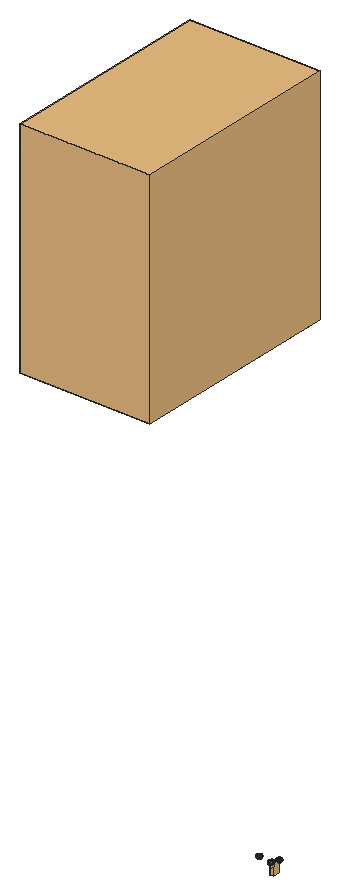
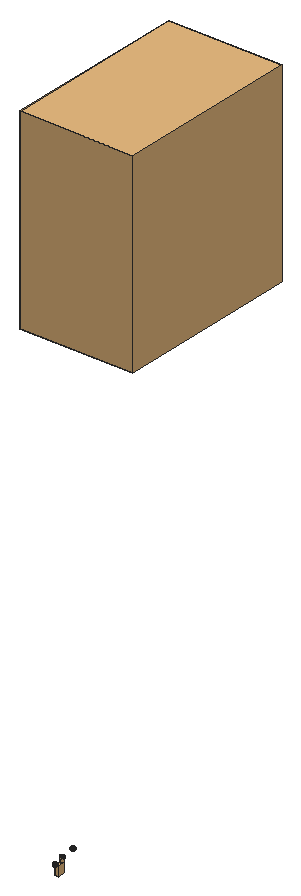
# SketchUp Ruby script. Lengths in inches.
U = 1.inch
M = Sketchup.active_model
def pt(a) = Geom::Point3d.new(a.map { |v| v * U })
def face(e, loops, mat)
  f = e.add_face(loops[0].map { |a| pt(a) })
  loops[1..].each { |l| e.add_face(l.map { |a| pt(a) }).erase! }
  f.material = f.back_material = mat if mat
  f
end
# faces: each face lists its corners as indices into pts; further lists are holes
def faces(e, pts, list, mat = nil) = list.each { |f| face(e, (f[0].is_a?(Array) ? f : [f]).map { |l| l.map { |i| pts[i] } }, mat) }
# xy, xz, yz: faces in a plane at the given z, y or x. An outline is a flat list of corners, or four numbers for a rectangle; further outlines are holes
def ring(l) = l.size == 4 ? [[l[0], l[1]], [l[2], l[1]], [l[2], l[3]], [l[0], l[3]]] : l.each_slice(2).to_a
def flat(e, list, mat, &to3) = list.each { |f| face(e, (f[0].is_a?(Array) ? f : [f]).map { |l| ring(l).map { |u, v| to3.(u, v) } }, mat) }
def xy(e, z, list, mat = nil) = flat(e, list, mat) { |x, y| [x, y, z] }
def xz(e, y, list, mat = nil) = flat(e, list, mat) { |x, z| [x, y, z] }
def yz(e, x, list, mat = nil) = flat(e, list, mat) { |y, z| [x, y, z] }
def lines(e, pts, list) = list.each { |a, b| e.add_line(pt(pts[a]), pt(pts[b])) }
# prism: a flat outline (further loops are holes) pulled along v
def prism(e, loops, v, mat = nil)
  f = face(e, loops, mat); d = Geom::Vector3d.new(v.map { |x| x * U })
  f.pushpull(f.normal.samedirection?(d) ? d.length : -d.length)
end
def box(e, o, s, mat = nil) = prism(e, [[o, [o[0] + s[0], o[1], o[2]], [o[0] + s[0], o[1] + s[1], o[2]], [o[0], o[1] + s[1], o[2]]]], [0, 0, s[2]], mat)
def at(x, y, z, deg = 0) = Geom::Transformation.translation(pt([x, y, z])) * Geom::Transformation.rotation(ORIGIN, Z_AXIS, deg.degrees)
def axes(o, x, y, z) = Geom::Transformation.new([*x, 0, *y, 0, *z, 0, *pt(o).to_a, 1])
def part(name) = M.definitions.add(name)
# library, detail: a bought-in or finely detailed component or shape, given as its bounding box
def library(name, o, s) = part(name).tap { |d| box(d.entities, o, s) }
def detail(e, o, s) = box(e.add_group.entities, o, s)
def put(e, d, t, mat = nil) = e.add_instance(d, t).tap { |i| i.material = mat if mat }
def group(e, t, mat = nil) = e.add_group.tap { |g| g.transformation = t; g.material = mat if mat }.entities
root = M.entities
M.materials.add("green").color = [174, 139, 102]
M.materials.add("vio").color = [206, 114, 100]
c1 = part("3DGeom~189_Defintion")
p = [[117.375,12.85,-489.11],[33.19,-268.35,-390.125],[-76.27,-85.37,-487.14],[256.79,-154.93,-392.4],[251.43,147.02,-400.02],[-53.49,177.1875,-454.76],
  [23.91,254.65,-403.32],[-199.3,-309.86,-283.32],[-277.61,-121.32,-394.64],[-165.29,120.48,-453.62],[-210.02,294.05,-298.55],[-281.54,99.72,-400.21],
  [46.16,332.12,-313.1],[-281.54,99.72,-400.21],[-277.61,-121.32,-394.64],[-432.71,-85.37,-236.39],[-281.54,99.72,-400.21],[-371.08,120.48,-308.85],
  [-371.08,120.48,-308.85],[411.58,0,-289.54],[289.98,281.2,-243.75],[411.58,0,-289.54],[251.43,147.02,-400.02],[289.98,281.2,-243.75],
  [-277.61,-121.32,-394.64],[-199.3,-309.86,-283.32],[-378.39,-268.35,-100.59],[-277.61,-121.32,-394.64],[133.75,-379.42,-188.58],[327.4,-281.2,-190.55],
  [133.75,-379.42,-188.58],[411.58,0,-289.54],[327.4,-281.2,-190.55],[256.79,-154.93,-392.4],[33.19,-268.35,-390.125],[-67.59,-415.375,-96.08],
  [-199.3,-309.86,-283.32],[33.19,-268.35,-390.125],[133.75,-379.42,-188.58],[7.3125,388.83,-208.26],[289.98,281.2,-243.75],[46.16,332.12,-313.1],
  [46.16,332.12,-313.1],[-210.02,294.05,-298.55],[-500,12.85,-54.8],[-409.93,177.1875,-204.01],[-210.02,294.05,-298.55],[-387.68,254.65,-113.79],
  [-210.02,294.05,-298.55],[-387.68,254.65,-113.79],[-310.28,332.12,-62.35],[-210.02,294.05,-298.55],[-198.48,388.83,-63.49],[-210.02,294.05,-298.55],
  [-82.23,409.58,-116.9],[-210.02,294.05,-298.55],[-210.02,294.05,-298.55],[411.58,0,-289.54],[461.45,-147.02,-101.47],[327.4,-281.2,-190.55],
  [456.09,154.93,-109.09],[411.58,0,-289.54],[289.98,281.2,-243.75],[411.58,0,-289.54],[-199.3,-309.86,-283.32],[-222.6875,-379.42,62.16],
  [-199.3,-309.86,-283.32],[-222.6875,-379.42,62.16],[-378.39,-268.35,-100.59],[222.6875,379.42,-62.16],[289.98,281.2,-243.75],[222.6875,379.42,-62.16],
  [289.98,281.2,-243.75],[-456.09,-154.93,109.09],[-461.45,147.02,101.47],[-387.68,254.65,-113.79],[327.4,-281.2,-190.55],[198.48,-388.83,63.49],
  [327.4,-281.2,-190.55],[310.28,-332.12,62.35],[310.28,-332.12,62.35],[327.4,-281.2,-190.55],[82.23,-409.58,116.9],[67.59,415.375,96.08],
  [-387.68,254.65,-113.79],[-327.4,281.2,190.55],[-387.68,254.65,-113.79],[-327.4,281.2,190.55],[-310.28,332.12,-62.35],[500,-12.85,54.8],
  [378.39,268.35,100.59],[222.6875,379.42,-62.16],[387.68,-254.65,113.79],[310.28,-332.12,62.35],[-222.6875,-379.42,62.16],[-289.98,-281.2,243.75],
  [-7.3125,-388.83,208.26],[-222.6875,-379.42,62.16],[-133.75,379.42,188.58],[-327.4,281.2,190.55],[378.39,268.35,100.59],[-411.58,0,289.54],
  [409.93,-177.1875,204.01],[432.71,85.37,236.39],[-222.6875,-379.42,62.16],[-46.16,-332.12,313.1],[-222.6875,-379.42,62.16],[-46.16,-332.12,313.1],
  [-289.98,-281.2,243.75],[210.02,-294.05,298.55],[387.68,-254.65,113.79],[199.3,309.86,283.32],[378.39,268.35,100.59],[199.3,309.86,283.32],
  [-256.79,154.93,392.4],[-256.79,154.93,392.4],[-327.4,281.2,190.55],[-251.43,-147.02,400.02],[-251.43,-147.02,400.02],[210.02,-294.05,298.55],
  [-327.4,281.2,190.55],[-33.19,268.35,390.13],[-133.75,379.42,188.58],[-33.19,268.35,390.13],[-327.4,281.2,190.55],[-256.79,154.93,392.4],
  [-33.19,268.35,390.13],[371.08,-120.48,308.85],[210.02,-294.05,298.55],[-46.16,-332.12,313.1],[277.61,121.32,394.64],[199.3,309.86,283.32],
  [-289.98,-281.2,243.75],[-46.16,-332.12,313.1],[-23.91,-254.65,403.32],[-289.98,-281.2,243.75],[-251.43,-147.02,400.02],[-33.19,268.35,390.13],
  [277.61,121.32,394.64],[199.3,309.86,283.32],[-411.58,0,289.54],[-117.375,-12.85,489.11],[-411.58,0,289.54],[210.02,-294.05,298.55],
  [53.49,-177.1875,454.76],[210.02,-294.05,298.55],[165.29,-120.48,453.62],[210.02,-294.05,298.55],[281.54,-99.72,400.21],[210.02,-294.05,298.55],
  [371.08,-120.48,308.85],[281.54,-99.72,400.21],[210.02,-294.05,298.55],[281.54,-99.72,400.21],[76.27,85.37,487.14],[-33.19,268.35,390.13],
  [-33.19,268.35,390.13],[277.61,121.32,394.64],[281.54,-99.72,400.21],[277.61,121.32,394.64],[281.54,-99.72,400.21]]
faces(c1.entities,p,[[0,1,2],[0,3,1],[4,3,0],[5,0,2],[6,0,5],[6,4,0],[2,7,8],[2,1,7],
  [9,2,8],[5,2,9],[5,9,10],[6,5,10],[9,8,11],[9,11,10],[12,4,6],[12,6,10],
  [13,14,15],[16,15,17],[11,18,10],[4,19,3],[20,21,22],[12,23,4],[24,25,26],[27,26,15],
  [3,28,1],[3,29,30],[31,32,33],[34,35,36],[37,38,35],[39,40,41],[39,42,43],[17,15,44],
  [17,44,45],[17,45,46],[45,47,48],[49,50,51],[50,52,53],[54,39,55],[52,54,56],[57,58,59],
  [60,58,61],[62,60,63],[64,35,65],[66,67,68],[69,60,70],[39,71,72],[15,26,73],[15,73,44],
  [54,71,39],[45,44,74],[45,74,75],[76,77,38],[78,79,77],[58,80,81],[38,82,35],[38,77,82],
  [54,83,71],[52,83,54],[84,74,85],[86,87,88],[60,89,58],[90,89,60],[91,90,60],[58,92,93],
  [89,92,58],[26,94,95],[26,95,73],[35,96,97],[35,82,96],[50,98,52],[52,98,83],[50,99,98],
  [83,100,71],[44,73,101],[44,101,74],[89,102,92],[103,102,89],[90,103,89],[104,96,105],[106,107,108],
  [77,79,109],[79,110,109],[82,77,109],[83,111,112],[98,111,83],[113,103,90],[74,101,114],[74,115,116],
  [73,95,117],[73,118,101],[92,102,119],[96,82,109],[120,121,122],[98,123,111],[124,125,126],[102,127,128],
  [103,127,102],[129,96,109],[130,127,103],[131,130,103],[132,133,134],[135,134,136],[137,138,139],[140,136,141],
  [142,141,125],[134,133,143],[144,134,145],[146,144,147],[148,146,149],[150,151,152],[130,153,127],[125,154,155],
  [156,154,157],[125,141,154],[154,158,159],[136,134,144],[136,144,141],[154,146,160],[141,144,146],[141,146,154]],"vio")
c2 = library("plants1",[-17.48,-17.55,0],[53.57,32.72,56.26])
c3 = library("3DGeom~102_Defintion",[-331.46,-500,-168.38],[662.92,1000,336.76])
c4 = part("3DGeom~103_Defintion")
p = [[302.66,-500,-146.11],[317.99,-495.14,-154.33],[299.97,-497.07,-128.32],[317.99,-495.14,-154.33],[302.66,-500,-146.11],[309.56,-498.4,-152.34],
  [299.97,-497.07,-128.32],[317.99,-495.14,-154.33],[312.61,-489.29,-118.76],[312.61,-489.29,-118.76],[317.99,-495.14,-154.33],[327.95,-484.43,-126.98],
  [317.99,-495.14,-154.33],[325.71,-491.1,-151.56],[330.64,-487.36,-144.77],[327.95,-484.43,-126.98],[317.99,-495.14,-154.33],[330.64,-487.36,-144.77],
  [302.66,-500,-146.11],[299.97,-497.07,-128.32],[299.15,-499.51,-137.32],[327.95,-484.43,-126.98],[330.64,-487.36,-144.77],[331.46,-484.92,-135.77],
  [299.97,-497.07,-128.32],[312.61,-489.29,-118.76],[304.89,-493.33,-121.53],[312.61,-489.29,-118.76],[327.95,-484.43,-126.98],[321.05,-486.03,-120.75],
  [-317.36,495.99,133.65],[-331.46,484.07,150.24],[-328.26,482.74,159.03],[-317.36,495.99,133.65],[-328.26,482.74,159.03],[-321.59,483.72,165.67],
  [-317.36,495.99,133.65],[-321.59,483.72,165.67],[-313.24,486.75,168.38],[-317.36,495.99,133.65],[-330.32,487.36,141.66],[-331.46,484.07,150.24],
  [-317.36,495.99,133.65],[-313.24,486.75,168.38],[-305.4375,491.02,166.44],[-317.36,495.99,133.65],[-325.17,491.72,135.59],[-330.32,487.36,141.66],
  [-317.36,495.99,133.65],[-305.4375,491.02,166.44],[-300.28,495.38,160.37],[-317.36,495.99,133.65],[-300.28,495.38,160.37],[-299.15,498.67,151.79],
  [-317.36,495.99,133.65],[-299.15,498.67,151.79],[-302.34,500,143.01],[-317.36,495.99,133.65],[-302.34,500,143.01],[-309.01,499.02,136.36]]
faces(c4.entities,p,[[0,1,2],[3,4,5],[6,7,8],[9,10,11],[12,13,14],[15,16,17],[18,19,20],[21,22,23],
  [24,25,26],[27,28,29],[30,31,32],[33,34,35],[36,37,38],[39,40,41],[42,43,44],[45,46,47],
  [48,49,50],[51,52,53],[54,55,56],[57,58,59]],"green")
c5 = library("3DGeom~104_Defintion",[-334.52,-500,-160.51],[669.04,1000,321.02])
c6 = part("3DGeom~105_Defintion")
p = [[-306.36,-487.18,-90.84],[-301.3,-484.5,-160.51],[-278.52,-498.77,-106.98],[-278.52,-498.77,-106.98],[-301.3,-484.5,-160.51],[-275.99,-497.43,-141.8125],
  [-301.3,-484.5,-160.51],[-286.29,-491.76,-155.1],[-275.99,-497.43,-141.8125],[-331.67,-474.24,-109.53],[-301.3,-484.5,-160.51],[-306.36,-487.18,-90.84],
  [-329.14,-472.9,-144.36],[-301.3,-484.5,-160.51],[-331.67,-474.24,-109.53],[-301.3,-484.5,-160.51],[-329.14,-472.9,-144.36],[-316.98,-477.6,-156.58],
  [-329.14,-472.9,-144.36],[-331.67,-474.24,-109.53],[-334.52,-471.68,-127.14],[-278.52,-498.77,-106.98],[-275.99,-497.43,-141.8125],[-273.14,-500,-124.2],
  [-331.67,-474.24,-109.53],[-306.36,-487.18,-90.84],[-321.37,-479.92,-96.24],[-306.36,-487.18,-90.84],[-278.52,-498.77,-106.98],[-290.68,-494.08,-94.77],
  [313.125,494.74,102.45],[292.39,466.72,160.51],[309.13,461.51,157.36],[313.125,494.74,102.45],[309.13,461.51,157.36],[324.16,461.46,147.27],
  [313.125,494.74,102.45],[324.16,461.46,147.27],[333.45,466.57,132.95],[313.125,494.74,102.45],[333.45,466.57,132.95],[334.52,475.47,118.24],
  [313.125,494.74,102.45],[278.4375,475.68,155.88],[292.39,466.72,160.51],[313.125,494.74,102.45],[334.52,475.47,118.24],[327.08,485.78,107.08],
  [313.125,494.74,102.45],[271,485.99,144.72],[278.4375,475.68,155.88],[313.125,494.74,102.45],[272.07,494.89,130.01],[271,485.99,144.72],
  [313.125,494.74,102.45],[281.36,500,115.69],[272.07,494.89,130.01],[313.125,494.74,102.45],[296.39,499.94,105.61],[281.36,500,115.69]]
faces(c6.entities,p,[[0,1,2],[3,4,5],[6,7,8],[9,10,11],[12,13,14],[15,16,17],[18,19,20],[21,22,23],
  [24,25,26],[27,28,29],[30,31,32],[33,34,35],[36,37,38],[39,40,41],[42,43,44],[45,46,47],
  [48,49,50],[51,52,53],[54,55,56],[57,58,59]],"green")
c7 = part("3DGeom~222_Defintion")
p = [[138.17,-187.6,-427.375],[-199.9375,-99.75,-443.62],[24.02,0,-500],[340.4,-62.72,-359.51],[-304.37,62.72,-390.49],[340.4,-62.72,-359.51],
  [241.54,99.75,-422.41],[-96.57,187.6,-438.65],[-101.08,-262.21,-380.72],[-370.32,-172.76,-268.37],[-430.61,-78.97,-237.69],[-430.61,-78.97,-237.69],
  [-386.39,181.65,-235.57],[137.11,262.21,-369.28],[-386.39,181.65,-235.57],[-191.28,324.93,-259.77],[137.11,262.21,-369.28],[-191.28,324.93,-259.77],
  [215.3,-324.93,-240.23],[407.19,-181.65,-197.45],[407.19,-181.65,-197.45],[340.4,-62.72,-359.51],[451.41,78.97,-195.32],[340.4,-62.72,-359.51],
  [241.54,99.75,-422.41],[241.54,99.75,-422.41],[394.34,172.77,-231.63],[394.34,172.77,-231.63],[137.11,262.21,-369.28],[-304.37,62.72,-390.49],
  [-430.61,-78.97,-237.69],[-477.97,-10.3,-148.25],[-304.37,62.72,-390.49],[-386.39,181.65,-235.57],[-34.29,-381.14,-218.65],[-313.24,-266.5625,-232.06],
  [-101.08,-262.21,-380.72],[-34.29,-381.14,-218.65],[-313.24,-266.5625,-232.06],[394.34,172.77,-231.63],[137.11,262.21,-369.28],[334.05,266.5625,-200.96],
  [137.11,262.21,-369.28],[-191.28,324.93,-259.77],[55.09,381.14,-214.36],[334.05,266.5625,-200.96],[137.11,262.21,-369.28],[55.09,381.14,-214.36],
  [489.98,10.3,-101.75],[407.19,-181.65,-197.45],[-370.32,-172.76,-268.37],[-313.24,-266.5625,-232.06],[-441.48,-199.49,-21.21],[-370.32,-172.76,-268.37],
  [-191.28,324.93,-259.77],[-424.03,225.18,-20.37],[-191.28,324.93,-259.77],[-234.74,375.19,-11.28],[-191.28,324.93,-259.77],[-234.74,375.19,-11.28],
  [234.74,-375.19,11.28],[-34.29,-381.14,-218.65],[215.3,-324.93,-240.23],[424.03,-225.18,20.37],[234.74,-375.19,11.28],[215.3,-324.93,-240.23],
  [215.3,-324.93,-240.23],[-499.7,14.83,-24.01],[-34.29,-381.14,-218.65],[-274.68,-335.23,-138.48],[-313.24,-266.5625,-232.06],[-313.24,-266.5625,-232.06],
  [-274.68,-335.23,-138.48],[441.48,199.49,21.21],[334.05,266.5625,-200.96],[-17.45,-424.67,-0.84],[-34.29,-381.14,-218.65],[234.74,-375.19,11.28],
  [-34.29,-381.14,-218.65],[334.05,266.5625,-200.96],[286.69,335.23,-111.52],[286.69,335.23,-111.52],[17.45,424.67,0.84],[286.69,335.23,-111.52],
  [499.7,-14.83,24.01],[-264.96,-360.36,-12.73],[-274.68,-335.23,-138.48],[-264.96,-360.36,-12.73],[264.96,360.36,12.73],[286.69,335.23,-111.52],
  [264.96,360.36,12.73],[-489.98,-10.3,101.75],[-264.96,-360.36,-12.73],[-286.69,-335.23,111.52],[-286.69,-335.23,111.52],[-334.05,-266.5625,200.96],
  [-334.05,-266.5625,200.96],[-394.34,-172.77,231.63],[-451.41,-78.97,195.32],[-394.34,-172.77,231.63],[-407.19,181.65,197.45],[-234.74,375.19,-11.28],
  [-407.19,181.65,197.45],[-55.09,-381.14,214.36],[-286.69,-335.23,111.52],[-234.74,375.19,-11.28],[-407.19,181.65,197.45],[-215.3,324.93,240.23],
  [-215.3,324.93,240.23],[191.28,-324.93,259.77],[191.28,-324.93,259.77],[234.74,-375.19,11.28],[-215.3,324.93,240.23],[34.29,381.14,218.65],
  [264.96,360.36,12.73],[386.39,-181.65,235.57],[191.28,-324.93,259.77],[274.68,335.23,138.48],[264.96,360.36,12.73],[274.68,335.23,138.48],
  [477.97,10.3,148.25],[430.61,78.97,237.69],[370.32,172.77,268.37],[313.24,266.5625,232.06],[-407.19,181.65,197.45],[-137.11,-262.21,369.28],
  [-137.11,-262.21,369.28],[-334.05,-266.5625,200.96],[274.68,335.23,138.48],[101.08,262.21,380.72],[274.68,335.23,138.48],[101.08,262.21,380.72],
  [313.24,266.5625,232.06],[-340.4,62.72,359.51],[-394.34,-172.77,231.63],[-407.19,181.65,197.45],[-340.4,62.72,359.51],[-215.3,324.93,240.23],
  [-407.19,181.65,197.45],[-340.4,62.72,359.51],[-241.54,-99.75,422.41],[-394.34,-172.77,231.63],[-334.05,-266.5625,200.96],[-334.05,-266.5625,200.96],
  [-137.11,-262.21,369.28],[96.57,-187.6,438.65],[-55.09,-381.14,214.36],[-55.09,-381.14,214.36],[191.28,-324.93,259.77],[34.29,381.14,218.65],
  [-138.17,187.6,427.375],[34.29,381.14,218.65],[101.08,262.21,380.72],[-340.4,62.72,359.51],[-394.34,-172.77,231.63],[-241.54,-99.75,422.41],
  [313.24,266.5625,232.06],[199.9375,99.75,443.62],[313.24,266.5625,232.06],[370.32,172.77,268.37],[304.37,-62.72,390.49],[191.28,-324.93,259.77],
  [386.39,-181.65,235.57],[304.37,-62.72,390.49],[370.32,172.77,268.37],[304.37,-62.72,390.49],[430.61,78.97,237.69],[304.37,-62.72,390.49],
  [191.28,-324.93,259.77],[370.32,172.77,268.37],[304.37,-62.72,390.49],[-24.02,0,500],[304.37,-62.72,390.49]]
faces(c7.entities,p,[[0,1,2],[3,0,2],[2,1,4],[5,2,6],[2,4,7],[6,2,7],[8,9,1],[0,8,1],
  [1,9,10],[1,11,4],[7,4,12],[6,7,13],[7,14,15],[16,7,17],[18,8,0],[19,18,0],
  [20,0,21],[22,23,24],[22,25,26],[27,6,28],[29,30,31],[32,31,33],[34,35,36],[18,37,8],
  [8,38,9],[39,40,41],[42,43,44],[45,46,47],[48,49,23],[48,23,22],[50,51,52],[30,53,52],
  [54,33,55],[56,55,57],[47,58,59],[60,61,62],[63,64,65],[63,66,49],[31,30,52],[33,31,67],
  [33,67,55],[68,69,70],[71,72,52],[22,26,73],[26,74,73],[75,69,76],[77,75,78],[79,47,80],
  [81,47,82],[47,59,82],[74,83,73],[84,63,49],[84,49,48],[48,22,73],[67,31,52],[75,85,69],
  [86,87,52],[83,88,73],[89,82,90],[84,48,73],[91,67,52],[55,67,91],[92,93,52],[94,95,52],
  [96,97,52],[98,91,52],[99,98,52],[55,91,100],[101,55,102],[103,85,75],[103,104,85],[105,106,107],
  [82,59,108],[109,103,75],[110,75,111],[82,112,113],[114,82,113],[115,116,64],[115,64,63],[88,117,73],
  [118,113,119],[120,115,63],[120,63,84],[120,84,73],[121,120,73],[122,121,73],[123,122,73],[117,123,73],
  [124,91,98],[125,104,103],[126,127,104],[128,113,129],[130,131,132],[121,115,120],[133,98,134],[135,98,136],
  [137,138,139],[140,141,142],[140,143,144],[145,144,146],[145,147,148],[149,137,150],[151,150,152],[153,154,155],
  [156,152,157],[158,157,159],[160,161,162],[121,163,115],[164,165,166],[137,139,150],[167,145,168],[169,157,170],
  [150,139,140],[171,140,144],[171,144,145],[152,150,171],[152,171,157],[157,145,172],[150,140,171],[157,171,145]],"vio")
c8 = part("3DGeom~223_Defintion")
p = [[134.41,-263.08,-369.41],[-98.49,-186.72,-438.75],[24.02,0,-500],[240.51,-101.38,-422.46],[-198.9,101.38,-443.57],[240.51,-101.38,-422.46],
  [140.09,186.72,-427.28],[-98.38,263.08,-380.59],[-305,-60.32,-390.52],[-368.53,175.6,-268.28],[-310.49,268.95,-231.92],[-310.49,268.95,-231.92],
  [51.17,-381.46,-214.55],[-194.61,-323.41,-259.93],[51.17,-381.46,-214.55],[240.51,-101.38,-422.46],[341.03,60.32,-359.48],[341.03,60.32,-359.48],
  [218.625,323.41,-240.08],[-30.37,381.46,-218.47],[-30.37,381.46,-218.47],[218.625,323.41,-240.08],[331.3,-268.95,-201.09],[240.51,-101.38,-422.46],
  [331.3,-268.95,-201.09],[240.51,-101.38,-422.46],[392.55,-175.6,-231.72],[392.55,-175.6,-231.72],[240.51,-101.38,-422.46],[341.03,60.32,-359.48],
  [-388.24,-178.7,-235.66],[-388.24,-178.7,-235.66],[-429.78,82.24,-237.65],[-305,-60.32,-390.52],[-429.78,82.24,-237.65],[-98.38,263.08,-380.59],
  [-310.49,268.95,-231.92],[-271.23,337.3,-138.32],[-98.38,263.08,-380.59],[-30.37,381.46,-218.47],[283.24,-337.3,-111.68],[51.17,-381.46,-214.55],
  [134.41,-263.08,-369.41],[283.24,-337.3,-111.68],[134.41,-263.08,-369.41],[331.3,-268.95,-201.09],[450.59,-82.24,-195.36],[409.04,178.7,-197.36],
  [341.03,60.32,-359.48],[218.625,323.41,-240.08],[409.04,178.7,-197.36],[-368.53,175.6,-268.28],[-429.78,82.24,-237.65],[-439.41,202.76,-21.11],
  [-310.49,268.95,-231.92],[-368.53,175.6,-268.28],[13.09,-424.78,0.63],[-238.58,-373.4375,-11.46],[-194.61,-323.41,-259.93],[-194.61,-323.41,-259.93],
  [-238.58,-373.4375,-11.46],[-388.24,-178.7,-235.66],[-194.61,-323.41,-259.93],[218.625,323.41,-240.08],[238.58,373.4375,11.46],[218.625,323.41,-240.08],
  [-13.09,424.78,-0.63],[218.625,323.41,-240.08],[238.58,373.4375,11.46],[-388.24,-178.7,-235.66],[-477.84,13.89,-148.24],[-429.78,82.24,-237.65],
  [-429.78,82.24,-237.65],[-238.58,-373.4375,-11.46],[-426.32,-222.03,-20.48],[-388.24,-178.7,-235.66],[-388.24,-178.7,-235.66],[-271.23,337.3,-138.32],
  [-310.49,268.95,-231.92],[331.3,-268.95,-201.09],[439.41,-202.76,21.11],[-261.25,362.3125,-12.55],[261.25,-362.3125,12.55],[261.25,-362.3125,12.55],
  [283.24,-337.3,-111.68],[283.24,-337.3,-111.68],[489.85,-13.89,-101.76],[426.32,222.03,20.48],[-499.83,-11.125,-24.01],[-261.25,362.3125,-12.55],
  [-271.23,337.3,-138.32],[261.25,-362.3125,12.55],[499.83,11.125,24.01],[-409.04,-178.7,197.36],[-489.85,13.89,101.76],[-450.59,82.24,195.36],
  [-392.55,175.6,231.72],[-331.3,268.95,201.09],[-331.3,268.95,201.09],[-283.24,337.3,111.68],[-283.24,337.3,111.68],[-261.25,362.3125,-12.55],
  [-218.625,-323.41,240.08],[-238.58,-373.4375,-11.46],[-218.625,-323.41,240.08],[-283.24,337.3,111.68],[30.37,-381.46,218.47],[-218.625,-323.41,240.08],
  [-51.17,381.46,214.55],[238.58,373.4375,11.46],[-51.17,381.46,214.55],[271.23,-337.3,138.32],[271.23,-337.3,138.32],[261.25,-362.3125,12.55],
  [194.61,323.41,259.93],[238.58,373.4375,11.46],[-51.17,381.46,214.55],[194.61,323.41,259.93],[271.23,-337.3,138.32],[388.24,178.7,235.66],
  [194.61,323.41,259.93],[310.49,-268.95,231.92],[368.53,-175.6,268.28],[429.78,-82.24,237.65],[477.84,-13.89,148.24],[-341.03,-60.32,359.48],
  [-341.03,-60.32,359.48],[-51.17,381.46,214.55],[-331.3,268.95,201.09],[310.49,-268.95,231.92],[271.23,-337.3,138.32],[305,60.32,390.52],
  [305,60.32,390.52],[-240.51,101.38,422.46],[-341.03,-60.32,359.48],[-240.51,101.38,422.46],[-140.09,-186.72,427.28],[-409.04,-178.7,197.36],
  [-218.625,-323.41,240.08],[-341.03,-60.32,359.48],[-409.04,-178.7,197.36],[-134.41,263.08,369.41],[-331.3,268.95,201.09],[-392.55,175.6,231.72],
  [-51.17,381.46,214.55],[-331.3,268.95,201.09],[-134.41,263.08,369.41],[194.61,323.41,259.93],[-51.17,381.46,214.55],[98.38,-263.08,380.59],
  [-218.625,-323.41,240.08],[30.37,-381.46,218.47],[310.49,-268.95,231.92],[98.38,-263.08,380.59],[-392.55,175.6,231.72],[-240.51,101.38,422.46],
  [368.53,-175.6,268.28],[98.38,-263.08,380.59],[310.49,-268.95,231.92],[388.24,178.7,235.66],[98.49,186.72,438.74],[305,60.32,390.52],
  [388.24,178.7,235.66],[429.78,-82.24,237.65],[198.9,-101.38,443.57],[368.53,-175.6,268.28],[429.78,-82.24,237.65],[98.38,-263.08,380.59],
  [-218.625,-323.41,240.08],[368.53,-175.6,268.28],[98.38,-263.08,380.59],[-24.02,0,500],[98.38,-263.08,380.59]]
faces(c8.entities,p,[[0,1,2],[0,2,3],[1,4,2],[5,2,6],[2,4,7],[2,7,6],[1,8,4],[8,9,4],
  [4,9,10],[4,11,7],[12,13,1],[14,1,0],[13,8,1],[15,6,16],[17,6,18],[6,7,19],
  [6,20,21],[22,0,23],[24,25,26],[27,28,29],[13,30,8],[31,32,33],[8,34,9],[35,36,37],
  [38,37,39],[40,41,42],[43,44,45],[27,29,46],[46,29,47],[48,49,50],[51,52,53],[54,55,53],
  [56,57,58],[56,59,41],[60,61,62],[47,63,64],[65,39,66],[67,66,68],[69,70,71],[72,70,53],
  [73,74,75],[74,70,76],[77,78,53],[79,27,80],[27,46,80],[39,37,81],[39,81,66],[82,56,41],
  [83,41,84],[85,79,80],[46,47,86],[86,47,87],[47,64,87],[46,86,80],[74,88,70],[70,88,53],
  [89,90,53],[91,85,80],[86,92,80],[86,87,92],[93,88,74],[93,94,88],[88,94,53],[94,95,53],
  [95,96,53],[96,97,53],[98,99,53],[100,101,53],[102,74,103],[104,93,74],[66,81,105],[106,57,56],
  [106,107,57],[66,105,108],[109,66,110],[111,106,56],[112,56,113],[87,64,114],[115,116,117],[118,91,80],
  [92,87,119],[87,120,119],[121,118,80],[122,121,80],[123,122,80],[124,123,80],[92,124,80],[92,119,124],
  [125,94,93],[126,95,94],[127,105,128],[129,106,130],[124,131,123],[124,119,132],[133,95,134],[135,96,95],
  [136,137,138],[136,139,140],[141,142,143],[144,145,146],[147,148,141],[149,150,151],[152,153,106],[141,154,155],
  [156,157,158],[159,160,161],[162,147,160],[163,164,165],[166,161,164],[167,136,168],[147,141,160],[169,164,170],
  [171,139,136],[171,155,139],[160,141,155],[164,136,172],[161,171,164],[161,160,171],[160,155,171],[164,171,136]],"vio")
g1 = group(root,at(15.3125,134.49,26.21))
put(g1,c1,axes([3.75,-0.22,14.87],[0,0.00039,0],[0,0,-0.00039],[-0.00039,0,0]),"vio")
put(root,c2,axes([18.8,122.89,79.5],[0,0.3,0],[-0.3,0,0],[0,0,0.3]))
g2 = group(root,at(15.3125,134.49,26.21))
put(g2,c3,axes([4,0.92,13.7],[0,0.00081,0],[0,0,-0.00081],[-0.00081,0,0]),"green")
put(g2,c4,axes([4,0.92,13.7],[0,0.00081,0],[0,0,-0.00081],[-0.00081,0,0]),"green")
g3 = group(root,at(15.3125,134.49,26.21))
put(g3,c5,axes([4.1,0.53,14.11],[0,0.00042,0],[0,0,-0.00042],[-0.00042,0,0]),"green")
put(g3,c6,axes([4.1,0.53,14.11],[0,0.00042,0],[0,0,-0.00042],[-0.00042,0,0]),"green")
g4 = group(root,at(15.3125,134.49,26.21))
put(g4,c7,axes([4.12,1.2,14.13],[0,0.00039,0],[0,0,-0.00039],[-0.00039,0,0]),"vio")
g5 = group(root,at(15.3125,134.49,26.21))
put(g5,c8,axes([4.16,0.38,14.35],[0,0.00039,0],[0,0,-0.00039],[-0.00039,0,0]),"vio")
